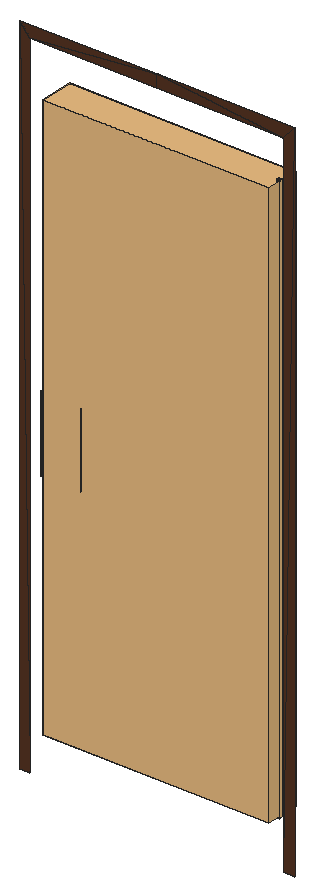
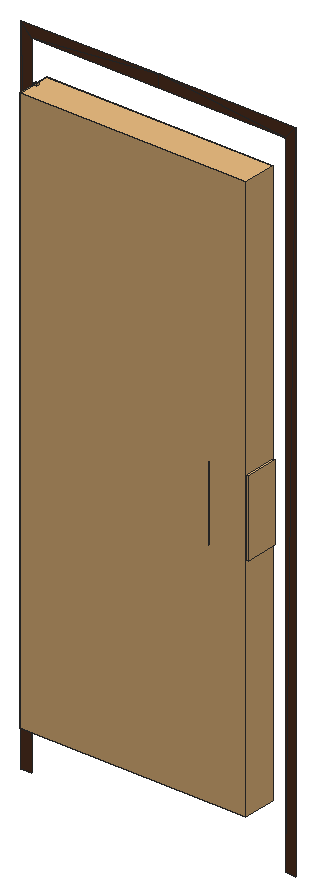
# SketchUp Ruby script. Lengths in inches.
U = 1.inch
M = Sketchup.active_model
def pt(a) = Geom::Point3d.new(a.map { |v| v * U })
def face(e, loops, mat)
  f = e.add_face(loops[0].map { |a| pt(a) })
  loops[1..].each { |l| e.add_face(l.map { |a| pt(a) }).erase! }
  f.material = f.back_material = mat if mat
  f
end
# faces: each face lists its corners as indices into pts; further lists are holes
def faces(e, pts, list, mat = nil) = list.each { |f| face(e, (f[0].is_a?(Array) ? f : [f]).map { |l| l.map { |i| pts[i] } }, mat) }
# xy, xz, yz: faces in a plane at the given z, y or x. An outline is a flat list of corners, or four numbers for a rectangle; further outlines are holes
def ring(l) = l.size == 4 ? [[l[0], l[1]], [l[2], l[1]], [l[2], l[3]], [l[0], l[3]]] : l.each_slice(2).to_a
def flat(e, list, mat, &to3) = list.each { |f| face(e, (f[0].is_a?(Array) ? f : [f]).map { |l| ring(l).map { |u, v| to3.(u, v) } }, mat) }
def xy(e, z, list, mat = nil) = flat(e, list, mat) { |x, y| [x, y, z] }
def xz(e, y, list, mat = nil) = flat(e, list, mat) { |x, z| [x, y, z] }
def yz(e, x, list, mat = nil) = flat(e, list, mat) { |y, z| [x, y, z] }
def lines(e, pts, list) = list.each { |a, b| e.add_line(pt(pts[a]), pt(pts[b])) }
# prism: a flat outline (further loops are holes) pulled along v
def prism(e, loops, v, mat = nil)
  f = face(e, loops, mat); d = Geom::Vector3d.new(v.map { |x| x * U })
  f.pushpull(f.normal.samedirection?(d) ? d.length : -d.length)
end
def box(e, o, s, mat = nil) = prism(e, [[o, [o[0] + s[0], o[1], o[2]], [o[0] + s[0], o[1] + s[1], o[2]], [o[0], o[1] + s[1], o[2]]]], [0, 0, s[2]], mat)
def at(x, y, z, deg = 0) = Geom::Transformation.translation(pt([x, y, z])) * Geom::Transformation.rotation(ORIGIN, Z_AXIS, deg.degrees)
def axes(o, x, y, z) = Geom::Transformation.new([*x, 0, *y, 0, *z, 0, *pt(o).to_a, 1])
def part(name) = M.definitions.add(name)
# library, detail: a bought-in or finely detailed component or shape, given as its bounding box
def library(name, o, s) = part(name).tap { |d| box(d.entities, o, s) }
def detail(e, o, s) = box(e.add_group.entities, o, s)
def put(e, d, t, mat = nil) = e.add_instance(d, t).tap { |i| i.material = mat if mat }
def group(e, t, mat = nil) = e.add_group.tap { |g| g.transformation = t; g.material = mat if mat }.entities
root = M.entities
M.materials.add("Material \#0").color = [86, 53, 35]
M.materials.add("Material \#1").color = [140, 140, 140]
c1 = library("3DGeom~9_Defintion",[456.52,-471.89,-18.89],[5.57,1000,5.49])
c2 = library("3DGeom~7_Defintion",[455.56,-471.94,-18.85],[5.55,1000,5.48])
c3 = part("3DGeom~8_Defintion")
xz(c3.entities,-471.94,[[458.125,-17.29,459.53,-16.11,457.73,-17.15],[458.125,-17.29,458.54,-17.29,459.53,-16.11],[458.54,-17.29,458.93,-17.15,459.53,-16.11],[457.73,-17.15,459.53,-16.11,457.42,-16.88],[458.93,-17.15,459.25,-16.88,459.53,-16.11],
  [457.42,-16.88,459.53,-16.11,457.21,-16.52],[459.25,-16.88,459.46,-16.52,459.53,-16.11],[457.21,-16.52,459.53,-16.11,457.14,-16.11],[457.14,-16.11,459.53,-16.11,457.21,-15.7],[459.53,-16.11,457.42,-15.34,457.21,-15.7],
  [459.53,-16.11,457.73,-15.07,457.42,-15.34],[459.53,-16.11,458.125,-14.93,457.73,-15.07],[459.53,-16.11,458.54,-14.93,458.125,-14.93],[459.53,-16.11,458.93,-15.07,458.54,-14.93],[459.53,-16.11,459.25,-15.34,458.93,-15.07],
  [459.53,-16.11,459.46,-15.7,459.25,-15.34]],"Material \#1")
xz(c3.entities,-416.39,[[458.125,-17.29,457.73,-17.15,459.53,-16.11],[458.125,-17.29,459.53,-16.11,458.54,-17.29],[458.54,-17.29,459.53,-16.11,458.93,-17.15],[457.73,-17.15,457.42,-16.88,459.53,-16.11],[458.93,-17.15,459.53,-16.11,459.25,-16.88],
  [457.42,-16.88,457.21,-16.52,459.53,-16.11],[459.25,-16.88,459.53,-16.11,459.46,-16.52],[457.21,-16.52,457.14,-16.11,459.53,-16.11],[457.14,-16.11,457.21,-15.7,459.53,-16.11],[459.53,-16.11,457.21,-15.7,457.42,-15.34],
  [459.53,-16.11,457.42,-15.34,457.73,-15.07],[459.53,-16.11,457.73,-15.07,458.125,-14.93],[459.53,-16.11,458.125,-14.93,458.54,-14.93],[459.53,-16.11,458.54,-14.93,458.93,-15.07],[459.53,-16.11,458.93,-15.07,459.25,-15.34],
  [459.53,-16.11,459.25,-15.34,459.46,-15.7]],"Material \#1")
xz(c3.entities,-27.5,[[458.125,-17.29,459.53,-16.11,457.73,-17.15],[458.125,-17.29,458.54,-17.29,459.53,-16.11],[458.54,-17.29,458.93,-17.15,459.53,-16.11],[457.73,-17.15,459.53,-16.11,457.42,-16.88],[458.93,-17.15,459.25,-16.88,459.53,-16.11],
  [457.42,-16.88,459.53,-16.11,457.21,-16.52],[459.25,-16.88,459.46,-16.52,459.53,-16.11],[457.21,-16.52,459.53,-16.11,457.14,-16.11],[457.14,-16.11,459.53,-16.11,457.21,-15.7],[459.53,-16.11,457.42,-15.34,457.21,-15.7],
  [459.53,-16.11,457.73,-15.07,457.42,-15.34],[459.53,-16.11,458.125,-14.93,457.73,-15.07],[459.53,-16.11,458.54,-14.93,458.125,-14.93],[459.53,-16.11,458.93,-15.07,458.54,-14.93],[459.53,-16.11,459.25,-15.34,458.93,-15.07],
  [459.53,-16.11,459.46,-15.7,459.25,-15.34]],"Material \#1")
xz(c3.entities,28.06,[[458.125,-17.29,457.73,-17.15,459.53,-16.11],[458.125,-17.29,459.53,-16.11,458.54,-17.29],[458.54,-17.29,459.53,-16.11,458.93,-17.15],[457.73,-17.15,457.42,-16.88,459.53,-16.11],[458.93,-17.15,459.53,-16.11,459.25,-16.88],
  [457.42,-16.88,457.21,-16.52,459.53,-16.11],[459.25,-16.88,459.53,-16.11,459.46,-16.52],[457.21,-16.52,457.14,-16.11,459.53,-16.11],[457.14,-16.11,457.21,-15.7,459.53,-16.11],[459.53,-16.11,457.21,-15.7,457.42,-15.34],
  [459.53,-16.11,457.42,-15.34,457.73,-15.07],[459.53,-16.11,457.73,-15.07,458.125,-14.93],[459.53,-16.11,458.125,-14.93,458.54,-14.93],[459.53,-16.11,458.54,-14.93,458.93,-15.07],[459.53,-16.11,458.93,-15.07,459.25,-15.34],
  [459.53,-16.11,459.25,-15.34,459.46,-15.7]],"Material \#1")
xz(c3.entities,472.5,[[458.125,-17.29,459.53,-16.11,457.73,-17.15],[458.125,-17.29,458.54,-17.29,459.53,-16.11],[458.54,-17.29,458.93,-17.15,459.53,-16.11],[457.73,-17.15,459.53,-16.11,457.42,-16.88],[458.93,-17.15,459.25,-16.88,459.53,-16.11],
  [457.42,-16.88,459.53,-16.11,457.21,-16.52],[459.25,-16.88,459.46,-16.52,459.53,-16.11],[457.21,-16.52,459.53,-16.11,457.14,-16.11],[457.14,-16.11,459.53,-16.11,457.21,-15.7],[459.53,-16.11,457.42,-15.34,457.21,-15.7],
  [459.53,-16.11,457.73,-15.07,457.42,-15.34],[459.53,-16.11,458.125,-14.93,457.73,-15.07],[459.53,-16.11,458.54,-14.93,458.125,-14.93],[459.53,-16.11,458.93,-15.07,458.54,-14.93],[459.53,-16.11,459.25,-15.34,458.93,-15.07],
  [459.53,-16.11,459.46,-15.7,459.25,-15.34]],"Material \#1")
xz(c3.entities,528.06,[[458.125,-17.29,457.73,-17.15,459.53,-16.11],[458.125,-17.29,459.53,-16.11,458.54,-17.29],[458.54,-17.29,459.53,-16.11,458.93,-17.15],[457.73,-17.15,457.42,-16.88,459.53,-16.11],[458.93,-17.15,459.53,-16.11,459.25,-16.88],
  [457.42,-16.88,457.21,-16.52,459.53,-16.11],[459.25,-16.88,459.53,-16.11,459.46,-16.52],[457.21,-16.52,457.14,-16.11,459.53,-16.11],[457.14,-16.11,457.21,-15.7,459.53,-16.11],[459.53,-16.11,457.21,-15.7,457.42,-15.34],
  [459.53,-16.11,457.42,-15.34,457.73,-15.07],[459.53,-16.11,457.73,-15.07,458.125,-14.93],[459.53,-16.11,458.125,-14.93,458.54,-14.93],[459.53,-16.11,458.54,-14.93,458.93,-15.07],[459.53,-16.11,458.93,-15.07,459.25,-15.34],
  [459.53,-16.11,459.25,-15.34,459.46,-15.7]],"Material \#1")
c4 = part("3DGeom~21_Defintion")
xy(c4.entities,73.08,[[-976.3,-241.71,23.7,-241.71,-976.3,-223.46],[23.7,-241.71,5.45,-223.46,-976.3,-223.46],[23.7,-241.71,23.7,0,5.45,-223.46],[5.45,-223.46,23.7,0,5.45,0],[23.7,0,23.7,241.71,5.45,223.46],
  [5.45,0,23.7,0,5.45,223.46],[-976.3,223.46,23.7,241.71,-976.3,241.71],[-976.3,223.46,5.45,223.46,23.7,241.71]],"Material \#0")
c5 = library("3DGeom~6_Defintion",[-5.59,-471.8,-48.03],[468.87,1000,73.72])
c6 = library("3DGeom~3_Defintion",[-83.33,-500,-350],[620.1,1000,533.33])
xy(root,18.91,[[128.43,116.3125,128.38,116.33,128.39,116.35],[128.43,116.3125,128.39,116.35,128.4375,116.33],[128.43,116.3125,128.4375,116.33,128.49,116.3125],[128.49,116.3125,128.4375,116.33,128.49,116.33],[128.49,116.3125,128.49,116.33,128.55,116.33],
  [128.38,116.33,128.34,116.37,128.35,116.375],[128.38,116.33,128.35,116.375,128.39,116.35],[128.49,116.33,128.54,116.35,128.55,116.33],[128.55,116.33,128.54,116.35,128.59,116.37],[128.54,116.35,128.58,116.375,128.59,116.37],
  [128.34,116.37,128.31,116.41,128.32,116.42],[128.34,116.37,128.32,116.42,128.35,116.375],[128.59,116.37,128.58,116.375,128.62,116.41],[128.58,116.375,128.6,116.42,128.62,116.41],[128.31,116.41,128.3,116.47,128.32,116.47],
  [128.31,116.41,128.32,116.47,128.32,116.42],[128.62,116.41,128.6,116.42,128.63,116.47],[128.6,116.42,128.61,116.47,128.63,116.47],[128.3,116.47,128.31,116.52,128.32,116.51],[128.3,116.47,128.32,116.51,128.32,116.47],
  [128.61,116.47,128.6,116.51,128.62,116.52],[128.61,116.47,128.62,116.52,128.63,116.47],[128.32,116.51,128.31,116.52,128.35,116.55],[128.6,116.51,128.58,116.55,128.59,116.5625],[128.6,116.51,128.59,116.5625,128.62,116.52],
  [128.31,116.52,128.34,116.5625,128.35,116.55],[128.35,116.55,128.34,116.5625,128.39,116.58],[128.58,116.55,128.54,116.58,128.55,116.6],[128.58,116.55,128.55,116.6,128.59,116.5625],[128.34,116.5625,128.38,116.6,128.39,116.58],
  [128.39,116.58,128.38,116.6,128.4375,116.6],[128.54,116.58,128.49,116.6,128.49,116.62],[128.54,116.58,128.49,116.62,128.55,116.6],[128.38,116.6,128.43,116.62,128.4375,116.6],[128.4375,116.6,128.43,116.62,128.49,116.6],
  [128.49,116.6,128.43,116.62,128.49,116.62]],"Material \#1")
xy(root,18.93,[[128.43,116.3125,128.4375,116.33,128.38,116.33],[128.43,116.3125,128.49,116.3125,128.49,116.33],[128.43,116.3125,128.49,116.33,128.4375,116.33],[128.49,116.3125,128.54,116.35,128.49,116.33],[128.49,116.3125,128.55,116.33,128.54,116.35],
  [128.38,116.33,128.39,116.35,128.34,116.37],[128.38,116.33,128.4375,116.33,128.39,116.35],[128.55,116.33,128.58,116.375,128.54,116.35],[128.55,116.33,128.59,116.37,128.58,116.375],[128.39,116.35,128.35,116.375,128.34,116.37],
  [128.34,116.37,128.35,116.375,128.31,116.41],[128.59,116.37,128.6,116.42,128.58,116.375],[128.59,116.37,128.62,116.41,128.6,116.42],[128.35,116.375,128.32,116.42,128.31,116.41],[128.31,116.41,128.32,116.42,128.3,116.47],
  [128.62,116.41,128.61,116.47,128.6,116.42],[128.62,116.41,128.63,116.47,128.61,116.47],[128.32,116.42,128.32,116.47,128.3,116.47],[128.3,116.47,128.32,116.47,128.31,116.52],[128.32,116.47,128.32,116.51,128.31,116.52],
  [128.61,116.47,128.63,116.47,128.6,116.51],[128.63,116.47,128.62,116.52,128.6,116.51],[128.32,116.51,128.34,116.5625,128.31,116.52],[128.32,116.51,128.35,116.55,128.34,116.5625],[128.6,116.51,128.62,116.52,128.58,116.55],
  [128.62,116.52,128.59,116.5625,128.58,116.55],[128.35,116.55,128.38,116.6,128.34,116.5625],[128.35,116.55,128.39,116.58,128.38,116.6],[128.58,116.55,128.59,116.5625,128.54,116.58],[128.59,116.5625,128.55,116.6,128.54,116.58],
  [128.39,116.58,128.43,116.62,128.38,116.6],[128.39,116.58,128.4375,116.6,128.43,116.62],[128.54,116.58,128.55,116.6,128.49,116.6],[128.4375,116.6,128.49,116.62,128.43,116.62],[128.4375,116.6,128.49,116.6,128.49,116.62],
  [128.49,116.6,128.55,116.6,128.49,116.62]],"Material \#1")
xy(root,22.4,[[128.43,116.3125,128.38,116.33,128.4375,116.33],[128.43,116.3125,128.4375,116.33,128.49,116.33],[128.43,116.3125,128.49,116.33,128.49,116.3125],[128.49,116.3125,128.49,116.33,128.54,116.35],[128.49,116.3125,128.54,116.35,128.55,116.33],
  [128.38,116.33,128.34,116.37,128.39,116.35],[128.38,116.33,128.39,116.35,128.4375,116.33],[128.55,116.33,128.54,116.35,128.58,116.375],[128.55,116.33,128.58,116.375,128.59,116.37],[128.39,116.35,128.34,116.37,128.35,116.375],
  [128.34,116.37,128.31,116.41,128.35,116.375],[128.59,116.37,128.58,116.375,128.6,116.42],[128.59,116.37,128.6,116.42,128.62,116.41],[128.35,116.375,128.31,116.41,128.32,116.42],[128.31,116.41,128.3,116.47,128.32,116.42],
  [128.62,116.41,128.6,116.42,128.61,116.47],[128.62,116.41,128.61,116.47,128.63,116.47],[128.32,116.42,128.3,116.47,128.32,116.47],[128.3,116.47,128.31,116.52,128.32,116.47],[128.32,116.47,128.31,116.52,128.32,116.51],
  [128.61,116.47,128.6,116.51,128.63,116.47],[128.63,116.47,128.6,116.51,128.62,116.52],[128.32,116.51,128.31,116.52,128.34,116.5625],[128.32,116.51,128.34,116.5625,128.35,116.55],[128.6,116.51,128.58,116.55,128.62,116.52],
  [128.62,116.52,128.58,116.55,128.59,116.5625],[128.35,116.55,128.34,116.5625,128.38,116.6],[128.35,116.55,128.38,116.6,128.39,116.58],[128.58,116.55,128.54,116.58,128.59,116.5625],[128.59,116.5625,128.54,116.58,128.55,116.6],
  [128.39,116.58,128.38,116.6,128.43,116.62],[128.39,116.58,128.43,116.62,128.4375,116.6],[128.54,116.58,128.49,116.6,128.55,116.6],[128.4375,116.6,128.43,116.62,128.49,116.62],[128.4375,116.6,128.49,116.62,128.49,116.6],
  [128.49,116.6,128.49,116.62,128.55,116.6]],"Material \#1")
xy(root,22.42,[[128.43,116.3125,128.39,116.35,128.38,116.33],[128.43,116.3125,128.4375,116.33,128.39,116.35],[128.43,116.3125,128.49,116.3125,128.4375,116.33],[128.49,116.3125,128.49,116.33,128.4375,116.33],[128.49,116.3125,128.55,116.33,128.49,116.33],
  [128.38,116.33,128.35,116.375,128.34,116.37],[128.38,116.33,128.39,116.35,128.35,116.375],[128.49,116.33,128.55,116.33,128.54,116.35],[128.55,116.33,128.59,116.37,128.54,116.35],[128.54,116.35,128.59,116.37,128.58,116.375],
  [128.34,116.37,128.32,116.42,128.31,116.41],[128.34,116.37,128.35,116.375,128.32,116.42],[128.59,116.37,128.62,116.41,128.58,116.375],[128.58,116.375,128.62,116.41,128.6,116.42],[128.31,116.41,128.32,116.47,128.3,116.47],
  [128.31,116.41,128.32,116.42,128.32,116.47],[128.62,116.41,128.63,116.47,128.6,116.42],[128.6,116.42,128.63,116.47,128.61,116.47],[128.3,116.47,128.32,116.47,128.32,116.51],[128.3,116.47,128.32,116.51,128.31,116.52],
  [128.61,116.47,128.62,116.52,128.6,116.51],[128.61,116.47,128.63,116.47,128.62,116.52],[128.32,116.51,128.35,116.55,128.31,116.52],[128.6,116.51,128.59,116.5625,128.58,116.55],[128.6,116.51,128.62,116.52,128.59,116.5625],
  [128.31,116.52,128.35,116.55,128.34,116.5625],[128.35,116.55,128.39,116.58,128.34,116.5625],[128.58,116.55,128.55,116.6,128.54,116.58],[128.58,116.55,128.59,116.5625,128.55,116.6],[128.34,116.5625,128.39,116.58,128.38,116.6],
  [128.39,116.58,128.4375,116.6,128.38,116.6],[128.54,116.58,128.49,116.62,128.49,116.6],[128.54,116.58,128.55,116.6,128.49,116.62],[128.38,116.6,128.4375,116.6,128.43,116.62],[128.4375,116.6,128.49,116.6,128.43,116.62],
  [128.49,116.6,128.49,116.62,128.43,116.62]],"Material \#1")
xz(root,115.85,[[101.89,47.41,101.88,47.42,101.92,47.52],[101.89,47.41,101.92,47.52,101.93,47.52]],"Material \#1")
xz(root,117.63,[[101.5,47.09,101.59,47.12,101.59,47.13],[101.59,47.12,101.68,47.18,101.59,47.13],[101.68,47.17,101.76,47.23,101.76,47.24],[101.76,47.23,101.82,47.32,101.76,47.24],[101.76,47.23,101.83,47.32,101.82,47.32],
  [101.82,47.32,101.83,47.32,101.88,47.42],[101.83,47.32,101.89,47.41,101.88,47.42],[101.56,47.37,101.5625,47.41,101.55,47.375],[101.56,47.37,101.57,47.4,101.5625,47.41],[101.57,47.4,101.57,47.44,101.5625,47.41],
  [101.57,47.4,101.58,47.44,101.57,47.44],[101.89,47.41,101.92,47.52,101.88,47.42],[101.89,47.41,101.93,47.52,101.92,47.52],[101.57,47.44,101.58,47.44,101.57,47.48],[101.58,47.44,101.58,47.48,101.57,47.48],
  [101.57,47.48,101.58,47.48,101.57,47.52],[101.58,47.48,101.58,47.52,101.57,47.52],[101.57,47.52,101.58,47.52,101.5625,47.56],[101.58,47.52,101.57,47.56,101.5625,47.56],[101.92,47.52,101.93,47.52,101.95,47.63],
  [101.93,47.52,101.96,47.63,101.95,47.63],[101.5625,47.56,101.57,47.56,101.55,47.59],[101.57,47.56,101.56,47.6,101.55,47.59],[101.95,47.63,101.96,47.63,101.96,47.76],[101.96,47.63,101.97,47.76,101.96,47.76],
  [101.96,47.76,101.97,47.76,101.96,53.83],[101.97,47.76,101.96,55.49,101.96,53.83],[101.97,47.76,101.97,55.49,101.96,55.49]],"Material \#1")
put(root,c1,axes([101.39,117.36,51.625],[0.05894,0,0],[0,0,0.06956],[0,0.05513,0]),"Material \#1")
put(root,c2,axes([101.39,117.36,51.625],[0.05906,0,0],[0,0,0.06971],[0,0.05524,0]),"Material \#1")
put(root,c3,axes([101.39,117.36,51.625],[0.05906,0,0],[0,0,0.06971],[0,0.05524,0]),"Material \#1")
put(root,c4,axes([113.53,121.22,92.68],[0,0,0.08171],[0.06923,0,0],[0,-0.06476,0]),"Material \#0")
put(root,c5,axes([101.39,117.36,51.625],[0.05875,0,0],[0,0,0.06934],[0,0.05495,0]),"Material \#1")
put(root,c6,axes([101.39,117.36,51.625],[0.00787,0,0],[0,0,0.00929],[0,0.00737,0]),"Material \#1")
